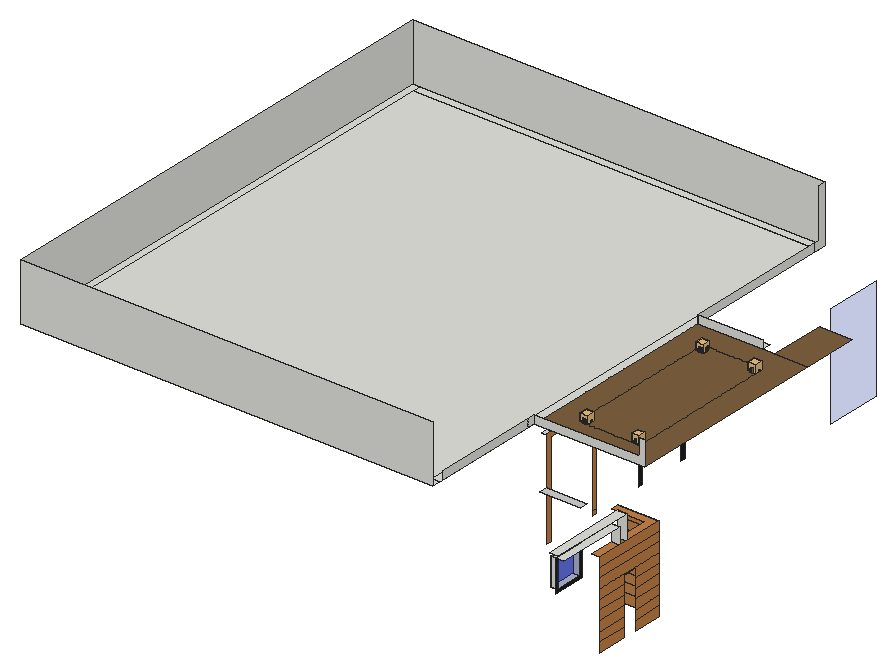
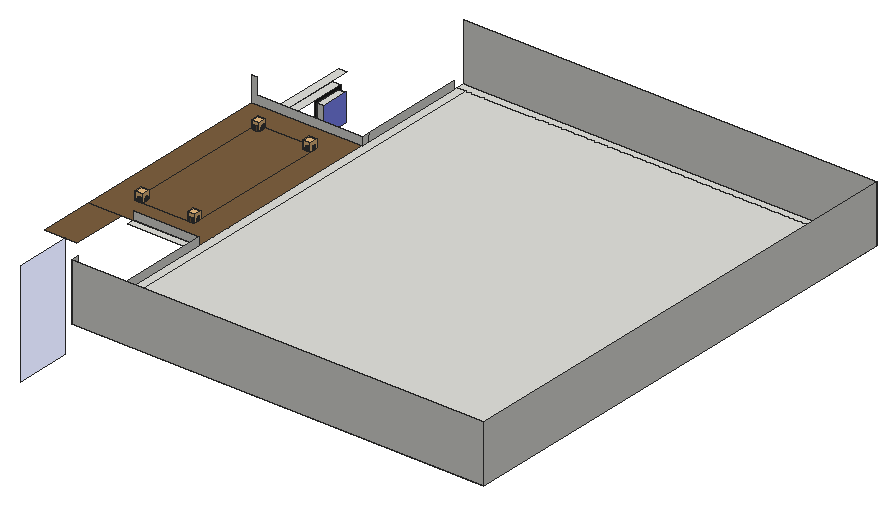
# SketchUp Ruby script. Lengths in inches.
U = 1.inch
M = Sketchup.active_model
def pt(a) = Geom::Point3d.new(a.map { |v| v * U })
def face(e, loops, mat)
  f = e.add_face(loops[0].map { |a| pt(a) })
  loops[1..].each { |l| e.add_face(l.map { |a| pt(a) }).erase! }
  f.material = f.back_material = mat if mat
  f
end
# faces: each face lists its corners as indices into pts; further lists are holes
def faces(e, pts, list, mat = nil) = list.each { |f| face(e, (f[0].is_a?(Array) ? f : [f]).map { |l| l.map { |i| pts[i] } }, mat) }
# xy, xz, yz: faces in a plane at the given z, y or x. An outline is a flat list of corners, or four numbers for a rectangle; further outlines are holes
def ring(l) = l.size == 4 ? [[l[0], l[1]], [l[2], l[1]], [l[2], l[3]], [l[0], l[3]]] : l.each_slice(2).to_a
def flat(e, list, mat, &to3) = list.each { |f| face(e, (f[0].is_a?(Array) ? f : [f]).map { |l| ring(l).map { |u, v| to3.(u, v) } }, mat) }
def xy(e, z, list, mat = nil) = flat(e, list, mat) { |x, y| [x, y, z] }
def xz(e, y, list, mat = nil) = flat(e, list, mat) { |x, z| [x, y, z] }
def yz(e, x, list, mat = nil) = flat(e, list, mat) { |y, z| [x, y, z] }
def lines(e, pts, list) = list.each { |a, b| e.add_line(pt(pts[a]), pt(pts[b])) }
# prism: a flat outline (further loops are holes) pulled along v
def prism(e, loops, v, mat = nil)
  f = face(e, loops, mat); d = Geom::Vector3d.new(v.map { |x| x * U })
  f.pushpull(f.normal.samedirection?(d) ? d.length : -d.length)
end
def box(e, o, s, mat = nil) = prism(e, [[o, [o[0] + s[0], o[1], o[2]], [o[0] + s[0], o[1] + s[1], o[2]], [o[0], o[1] + s[1], o[2]]]], [0, 0, s[2]], mat)
def at(x, y, z, deg = 0) = Geom::Transformation.translation(pt([x, y, z])) * Geom::Transformation.rotation(ORIGIN, Z_AXIS, deg.degrees)
def axes(o, x, y, z) = Geom::Transformation.new([*x, 0, *y, 0, *z, 0, *pt(o).to_a, 1])
def part(name) = M.definitions.add(name)
# library, detail: a bought-in or finely detailed component or shape, given as its bounding box
def library(name, o, s) = part(name).tap { |d| box(d.entities, o, s) }
def detail(e, o, s) = box(e.add_group.entities, o, s)
def put(e, d, t, mat = nil) = e.add_instance(d, t).tap { |i| i.material = mat if mat }
def group(e, t, mat = nil) = e.add_group.tap { |g| g.transformation = t; g.material = mat if mat }.entities
root = M.entities
M.materials.add("Glass_Basic_01").color = [23, 48, 186]
M.materials["Glass_Basic_01"].alpha = 0.25
M.materials.add("I03_Bluebell_Mist").color = [130, 140, 255]
M.materials.add("M08_Obsidian_Black").color = [30, 30, 30]
M.materials.add("Plywood_01_1K").color = [125, 96, 64]
M.materials.add("Wood_Floor_01_1K").color = [196, 130, 70]
M.materials.add("[Cladding_Siding_White]1").color = [207, 207, 207]
c1 = library("Sphere Light\#1",[-2.87,-2.87,-2.87],[5.74,5.74,5.74])
c2 = library("Sphere Light\#3",[-2.8,-2.8,-2.8],[5.6,5.6,5.6])
c3 = library("Sphere Light",[-2.75,-2.75,-2.75],[5.5,5.5,5.5])
c4 = library("Sphere Light\#2",[-2.64,-2.64,-2.64],[5.28,5.28,5.28])
xy(root,338.4,[[384,66.6,390,69],[384,69,390,77.4]],"Wood_Floor_01_1K")
xy(root,350,[[378.55,14,384,34]])
xy(root,357,[[312,87,342,93]],"[Cladding_Siding_White]1")
xy(root,360,[[384,45,390,63],[384,69,390,69,390,99,360,99,360,93,384,93]],"Wood_Floor_01_1K")
xy(root,370,[[378.55,14,384,34]])
xy(root,372,[[384,12,390,63]])
xy(root,378,[[384,6,390,69]])
xy(root,381,[[297,108,303,147],[297,150,303,189],[297,192,303,228]])
xy(root,396,[[0,0,6,360],[6,0,303,6],[6,6,297,354],[297,6,303,351],[303,243,351,249],
  [297,351,303,354],[6,354,303,360]])
xy(root,396,[[[303,93,384,243],[321,111,366,225]],[[321,111,366,225],[362.36,111.38,363.14,111.45,363.88,111.73,364.52,112.18,365.01,112.78,365.34,113.5,365.47,114.27,365.4,115.05,365.125,115.78,364.67,116.42,364.07,116.92,363.36,117.25,362.58,117.375,361.8,117.3,361.07,117.03,360.43,116.58,359.93,115.97,359.61,115.26,359.48,114.49,359.55,113.71,359.82,112.97,360.28,112.34,360.88,111.84,361.59,111.51],[324.58,111.38,325.36,111.45,326.09,111.73,326.73,112.18,327.23,112.78,327.56,113.5,327.6875,114.27,327.61,115.05,327.34,115.78,326.89,116.42,326.28,116.92,325.57,117.25,324.8,117.375,324.02,117.3,323.28,117.03,322.65,116.58,322.15,115.97,321.82,115.26,321.69,114.49,321.76,113.71,322.04,112.97,322.49,112.34,323.09,111.84,323.81,111.51],[324.58,217.96,325.36,218.03,326.09,218.31,326.73,218.76,327.23,219.36,327.56,220.08,327.6875,220.85,327.61,221.63,327.34,222.36,326.89,223,326.28,223.5,325.57,223.83,324.8,223.96,324.02,223.88,323.28,223.61,322.65,223.16,322.15,222.55,321.82,221.84,321.69,221.07,321.76,220.29,322.04,219.56,322.49,218.92,323.09,218.42,323.81,218.09],[362.36,217.96,363.14,218.03,363.88,218.31,364.52,218.76,365.01,219.36,365.34,220.08,365.47,220.85,365.4,221.63,365.125,222.36,364.67,223,364.07,223.5,363.36,223.83,362.58,223.96,361.8,223.88,361.07,223.61,360.43,223.16,359.93,222.55,359.61,221.84,359.48,221.07,359.55,220.29,359.82,219.56,360.28,218.92,360.88,218.42,361.59,218.09]],[360,243,384,283.95]],"Plywood_01_1K")
xy(root,399,[[324.58,111.38,323.81,111.51,323.09,111.84,322.49,112.34,322.04,112.97,321.76,113.71,321.69,114.49,321.82,115.26,322.15,115.97,322.65,116.58,323.28,117.03,324.02,117.3,324.8,117.375,325.57,117.25,326.28,116.92,326.89,116.42,327.34,115.78,327.61,115.05,327.6875,114.27,327.56,113.5,327.23,112.78,326.73,112.18,326.09,111.73,325.36,111.45],[362.36,111.38,361.59,111.51,360.88,111.84,360.28,112.34,359.82,112.97,359.55,113.71,359.48,114.49,359.61,115.26,359.93,115.97,360.43,116.58,361.07,117.03,361.8,117.3,362.58,117.375,363.36,117.25,364.07,116.92,364.67,116.42,365.125,115.78,365.4,115.05,365.47,114.27,365.34,113.5,365.01,112.78,364.52,112.18,363.88,111.73,363.14,111.45],[324.58,217.96,323.81,218.09,323.09,218.42,322.49,218.92,322.04,219.56,321.76,220.29,321.69,221.07,321.82,221.84,322.15,222.55,322.65,223.16,323.28,223.61,324.02,223.88,324.8,223.96,325.57,223.83,326.28,223.5,326.89,223,327.34,222.36,327.61,221.63,327.6875,220.85,327.56,220.08,327.23,219.36,326.73,218.76,326.09,218.31,325.36,218.03],[362.36,217.96,361.59,218.09,360.88,218.42,360.28,218.92,359.82,219.56,359.55,220.29,359.48,221.07,359.61,221.84,359.93,222.55,360.43,223.16,361.07,223.61,361.8,223.88,362.58,223.96,363.36,223.83,364.07,223.5,364.67,223,365.125,222.36,365.4,221.63,365.47,220.85,365.34,220.08,365.01,219.36,364.52,218.76,363.88,218.31,363.14,218.03]],"Plywood_01_1K")
xz(root,0,[[0,396,303,438]])
xz(root,14,[[378.55,350,384,370]])
xz(root,34,[[378.55,350,384,370]])
xz(root,63,[[384,360,390,372]])
xz(root,69,[[384,360,390,378]])
xz(root,93,[[303,396,303,402,381,402,381,414,384,414,384,396]])
xz(root,99,[[360,297,381,304],[381,297,390,304],[360,304,381,311],[381,304,390,311],[360,311,390,318],
  [360,318,390,325],[360,325,390,332],[360,332,390,339],[360,339,390,346],[360,346,390,353],
  [360,353,390,360]],"Wood_Floor_01_1K")
xz(root,243,[[303,396,351,402]])
xz(root,360,[[0,396,303,438]])
yz(root,0,[[0,396,360,438]])
yz(root,303,[[9,396,87,402],[87,396,93,402],[243,396,351,402],[351,396,360,396,360,438,354,438,354,402,351,402]])
yz(root,303,[[189,312,192,315],[228,312,231,312,231,384,189,384,189,381,228,381],[189,315,192,381]],"M08_Obsidian_Black")
yz(root,303,[[105,312,108,312,108,381,189,381,189,384,105,384],[147,312,150,315],[147,315,150,381]],"Wood_Floor_01_1K")
yz(root,360,[[294,327,336,403.5]],"Glass_Basic_01")
yz(root,378.55,[[14,350,34,370]],"I03_Bluebell_Mist")
yz(root,384,[[14,350,34,370]],"Glass_Basic_01")
yz(root,384,[[[12,348,36,372],[14,350,34,370]]],"M08_Obsidian_Black")
yz(root,390,[[45,297,66.6,304],[77.4,297,99,304],[45,304,66.6,311],[77.4,304,99,311],[45,311,66.6,318],
  [77.4,311,99,318],[45,318,66.6,325],[77.4,318,99,325],[45,325,66.6,332],[77.4,325,99,332],
  [45,332,66.6,332,66.6,338.4,77.4,338.4,77.4,332,99,332,99,339,45,339],[45,339,99,346],[45,346,99,353],[45,353,99,360]],"Wood_Floor_01_1K")
p = [[324.58,111.38,396],[323.81,111.51,396],[323.81,111.51,399],[324.58,111.38,399],[325.36,111.45,396],[325.36,111.45,399],
  [362.36,111.38,396],[361.59,111.51,396],[361.59,111.51,399],[362.36,111.38,399],[363.14,111.45,396],[363.14,111.45,399],
  [323.09,111.84,396],[323.09,111.84,399],[326.09,111.73,396],[326.09,111.73,399],[360.88,111.84,396],[360.88,111.84,399],
  [363.88,111.73,396],[363.88,111.73,399],[326.73,112.18,396],[326.73,112.18,399],[364.52,112.18,396],[364.52,112.18,399],
  [322.49,112.34,396],[322.49,112.34,399],[360.28,112.34,396],[360.28,112.34,399],[327.23,112.78,396],[327.23,112.78,399],
  [365.01,112.78,396],[365.01,112.78,399],[322.04,112.97,396],[322.04,112.97,399],[359.82,112.97,396],[359.82,112.97,399],
  [327.56,113.5,396],[327.56,113.5,399],[365.34,113.5,396],[365.34,113.5,399],[321.76,113.71,396],[321.76,113.71,399],
  [359.55,113.71,396],[359.55,113.71,399],[327.6875,114.27,396],[327.6875,114.27,399],[365.47,114.27,396],[365.47,114.27,399],
  [321.69,114.49,396],[321.69,114.49,399],[359.48,114.49,396],[359.48,114.49,399],[327.61,115.05,396],[327.61,115.05,399],
  [365.4,115.05,396],[365.4,115.05,399],[321.82,115.26,396],[321.82,115.26,399],[359.61,115.26,396],[359.61,115.26,399],
  [327.34,115.78,396],[327.34,115.78,399],[365.125,115.78,396],[365.125,115.78,399],[322.15,115.97,396],[322.15,115.97,399],
  [359.93,115.97,396],[359.93,115.97,399],[326.89,116.42,396],[326.89,116.42,399],[364.67,116.42,396],[364.67,116.42,399],
  [322.65,116.58,396],[322.65,116.58,399],[360.43,116.58,396],[360.43,116.58,399],[326.28,116.92,396],[326.28,116.92,399],
  [364.07,116.92,396],[364.07,116.92,399],[323.28,117.03,396],[323.28,117.03,399],[361.07,117.03,396],[361.07,117.03,399],
  [325.57,117.25,396],[325.57,117.25,399],[363.36,117.25,396],[363.36,117.25,399],[324.02,117.3,396],[324.02,117.3,399],
  [361.8,117.3,396],[361.8,117.3,399],[324.8,117.375,396],[324.8,117.375,399],[362.58,117.375,396],[362.58,117.375,399],
  [324.58,217.96,396],[323.81,218.09,396],[323.81,218.09,399],[324.58,217.96,399],[325.36,218.03,396],[325.36,218.03,399],
  [326.09,218.31,396],[326.09,218.31,399],[362.36,217.96,396],[361.59,218.09,396],[361.59,218.09,399],[362.36,217.96,399],
  [363.14,218.03,396],[363.14,218.03,399],[363.88,218.31,396],[363.88,218.31,399],[323.09,218.42,396],[323.09,218.42,399],
  [360.88,218.42,396],[360.88,218.42,399],[326.73,218.76,396],[326.73,218.76,399],[364.52,218.76,396],[364.52,218.76,399],
  [322.49,218.92,396],[322.49,218.92,399],[360.28,218.92,396],[360.28,218.92,399],[327.23,219.36,396],[327.23,219.36,399],
  [365.01,219.36,396],[365.01,219.36,399],[322.04,219.56,396],[322.04,219.56,399],[359.82,219.56,396],[359.82,219.56,399],
  [327.56,220.08,396],[327.56,220.08,399],[365.34,220.08,396],[365.34,220.08,399],[321.76,220.29,396],[321.76,220.29,399],
  [359.55,220.29,396],[359.55,220.29,399],[327.6875,220.85,396],[327.6875,220.85,399],[365.47,220.85,396],[365.47,220.85,399],
  [321.69,221.07,396],[321.69,221.07,399],[359.48,221.07,396],[359.48,221.07,399],[327.61,221.63,396],[327.61,221.63,399],
  [365.4,221.63,396],[365.4,221.63,399],[321.82,221.84,396],[321.82,221.84,399],[359.61,221.84,396],[359.61,221.84,399],
  [327.34,222.36,396],[327.34,222.36,399],[365.125,222.36,396],[365.125,222.36,399],[322.15,222.55,396],[322.15,222.55,399],
  [359.93,222.55,396],[359.93,222.55,399],[326.89,223,396],[326.89,223,399],[364.67,223,396],[364.67,223,399],
  [322.65,223.16,396],[322.65,223.16,399],[360.43,223.16,396],[360.43,223.16,399],[326.28,223.5,396],[326.28,223.5,399],
  [364.07,223.5,396],[364.07,223.5,399],[323.28,223.61,396],[323.28,223.61,399],[361.07,223.61,396],[361.07,223.61,399],
  [325.57,223.83,396],[325.57,223.83,399],[363.36,223.83,396],[363.36,223.83,399],[324.02,223.88,396],[324.02,223.88,399],
  [361.8,223.88,396],[361.8,223.88,399],[324.8,223.96,396],[324.8,223.96,399],[362.58,223.96,396],[362.58,223.96,399],
  [303,189,312],[303,189,315],[303,189,384]]
faces(root,p,[[0,1,2,3],[4,0,3,5],[6,7,8,9],[10,6,9,11],[1,12,13,2],[14,4,5,15],[7,16,17,8],[18,10,11,19],
  [20,14,15,21],[22,18,19,23],[12,24,25,13],[16,26,27,17],[28,20,21,29],[30,22,23,31],[24,32,33,25],[26,34,35,27],
  [36,28,29,37],[38,30,31,39],[32,40,41,33],[34,42,43,35],[44,36,37,45],[46,38,39,47],[40,48,49,41],[42,50,51,43],
  [52,44,45,53],[54,46,47,55],[48,56,57,49],[50,58,59,51],[60,52,53,61],[62,54,55,63],[56,64,65,57],[58,66,67,59],
  [68,60,61,69],[70,62,63,71],[64,72,73,65],[66,74,75,67],[76,68,69,77],[78,70,71,79],[72,80,81,73],[74,82,83,75],
  [84,76,77,85],[86,78,79,87],[80,88,89,81],[82,90,91,83],[92,84,85,93],[94,86,87,95],[88,92,93,89],[90,94,95,91],
  [96,97,98,99],[100,96,99,101],[102,100,101,103],[104,105,106,107],[108,104,107,109],[110,108,109,111],[97,112,113,98],[105,114,115,106],
  [116,102,103,117],[118,110,111,119],[112,120,121,113],[114,122,123,115],[124,116,117,125],[126,118,119,127],[120,128,129,121],[122,130,131,123],
  [132,124,125,133],[134,126,127,135],[128,136,137,129],[130,138,139,131],[140,132,133,141],[142,134,135,143],[136,144,145,137],[138,146,147,139],
  [148,140,141,149],[150,142,143,151],[144,152,153,145],[146,154,155,147],[156,148,149,157],[158,150,151,159],[152,160,161,153],[154,162,163,155],
  [164,156,157,165],[166,158,159,167],[160,168,169,161],[162,170,171,163],[172,164,165,173],[174,166,167,175],[168,176,177,169],[170,178,179,171],
  [180,172,173,181],[182,174,175,183],[176,184,185,177],[178,186,187,179],[188,180,181,189],[190,182,183,191],[184,188,189,185],[186,190,191,187]],"Plywood_01_1K")
lines(root,p,[[192,193],[193,194]])
put(root,c1,at(362.64,221.05,399))
put(root,c2,at(324.88,114.36,399))
put(root,c3,at(362.6,114.1875,399))
put(root,c4,at(324.51,220.95,399))
